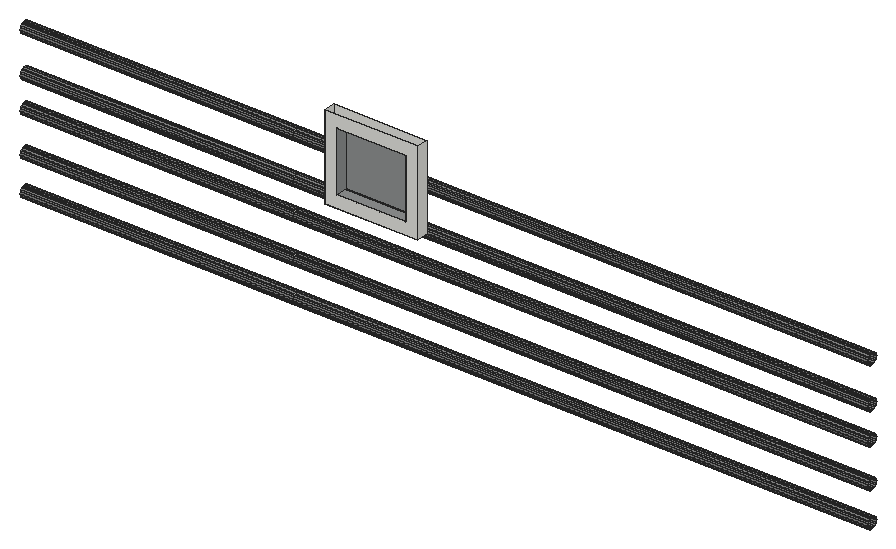
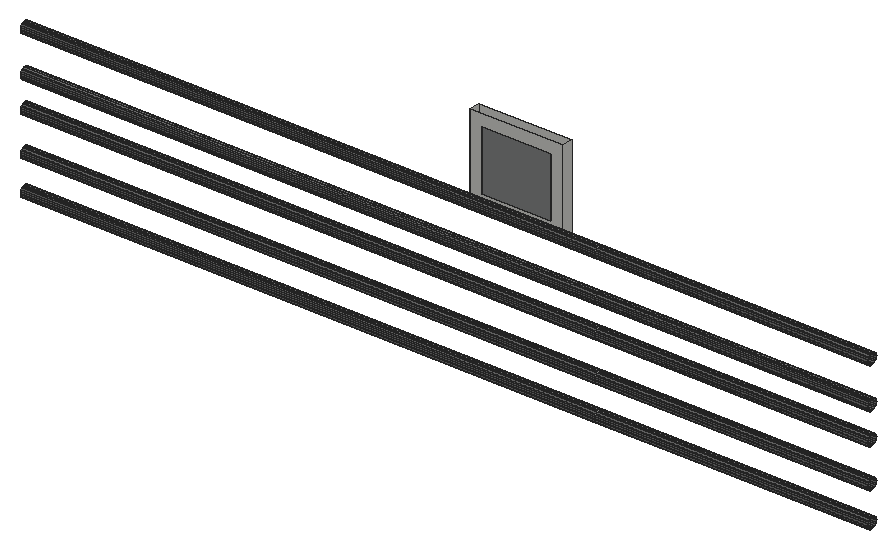
# SketchUp Ruby script. Lengths in inches.
U = 1.inch
M = Sketchup.active_model
def pt(a) = Geom::Point3d.new(a.map { |v| v * U })
def face(e, loops, mat)
  f = e.add_face(loops[0].map { |a| pt(a) })
  loops[1..].each { |l| e.add_face(l.map { |a| pt(a) }).erase! }
  f.material = f.back_material = mat if mat
  f
end
# faces: each face lists its corners as indices into pts; further lists are holes
def faces(e, pts, list, mat = nil) = list.each { |f| face(e, (f[0].is_a?(Array) ? f : [f]).map { |l| l.map { |i| pts[i] } }, mat) }
# xy, xz, yz: faces in a plane at the given z, y or x. An outline is a flat list of corners, or four numbers for a rectangle; further outlines are holes
def ring(l) = l.size == 4 ? [[l[0], l[1]], [l[2], l[1]], [l[2], l[3]], [l[0], l[3]]] : l.each_slice(2).to_a
def flat(e, list, mat, &to3) = list.each { |f| face(e, (f[0].is_a?(Array) ? f : [f]).map { |l| ring(l).map { |u, v| to3.(u, v) } }, mat) }
def xy(e, z, list, mat = nil) = flat(e, list, mat) { |x, y| [x, y, z] }
def xz(e, y, list, mat = nil) = flat(e, list, mat) { |x, z| [x, y, z] }
def yz(e, x, list, mat = nil) = flat(e, list, mat) { |y, z| [x, y, z] }
def lines(e, pts, list) = list.each { |a, b| e.add_line(pt(pts[a]), pt(pts[b])) }
# prism: a flat outline (further loops are holes) pulled along v
def prism(e, loops, v, mat = nil)
  f = face(e, loops, mat); d = Geom::Vector3d.new(v.map { |x| x * U })
  f.pushpull(f.normal.samedirection?(d) ? d.length : -d.length)
end
def box(e, o, s, mat = nil) = prism(e, [[o, [o[0] + s[0], o[1], o[2]], [o[0] + s[0], o[1] + s[1], o[2]], [o[0], o[1] + s[1], o[2]]]], [0, 0, s[2]], mat)
def at(x, y, z, deg = 0) = Geom::Transformation.translation(pt([x, y, z])) * Geom::Transformation.rotation(ORIGIN, Z_AXIS, deg.degrees)
def axes(o, x, y, z) = Geom::Transformation.new([*x, 0, *y, 0, *z, 0, *pt(o).to_a, 1])
def part(name) = M.definitions.add(name)
# library, detail: a bought-in or finely detailed component or shape, given as its bounding box
def library(name, o, s) = part(name).tap { |d| box(d.entities, o, s) }
def detail(e, o, s) = box(e.add_group.entities, o, s)
def put(e, d, t, mat = nil) = e.add_instance(d, t).tap { |i| i.material = mat if mat }
def group(e, t, mat = nil) = e.add_group.tap { |g| g.transformation = t; g.material = mat if mat }.entities
root = M.entities
M.materials.add("[0133_Gray]").color = [128, 128, 128]
M.materials.add("[Blacktop Old 02]").color = [143, 145, 145]
xy(root,158.26,[[226.04,223.92,236.29,225.17]])
xy(root,159.59,[[227.37,223.92,234.96,225.17]],"[Blacktop Old 02]")
xz(root,223.92,[[[226.04,158.26,236.29,167.57],[227.37,159.59,234.96,166.24]]])
xz(root,225.17,[[[226.04,158.26,236.29,167.57],[227.37,159.59,234.96,166.24]]])
xz(root,225.17,[[227.37,159.59,234.96,166.24]],"[Blacktop Old 02]")
yz(root,219.28,[[228.53,143.87,228.6875,143.89,228.84,143.95,228.97,144.05,229.07,144.18,229.13,144.33,229.15,144.49,229.13,144.66,229.07,144.81,228.97,144.9375,228.84,145.04,228.6875,145.1,228.53,145.12,228.36,145.1,228.21,145.04,228.08,144.9375,227.98,144.81,227.92,144.66,227.9,144.49,227.92,144.33,227.98,144.18,228.08,144.05,228.21,143.95,228.36,143.89],[228.53,147.74,228.6875,147.77,228.84,147.83,228.97,147.93,229.07,148.06,229.13,148.21,229.15,148.37,229.13,148.53,229.07,148.68,228.97,148.8125,228.84,148.91,228.6875,148.97,228.53,148.99,228.36,148.97,228.21,148.91,228.08,148.8125,227.98,148.68,227.92,148.53,227.9,148.37,227.92,148.21,227.98,148.06,228.08,147.93,228.21,147.83,228.36,147.77],[228.53,152.12,228.6875,152.14,228.84,152.2,228.97,152.3,229.07,152.43,229.13,152.58,229.15,152.74,229.13,152.91,229.07,153.06,228.97,153.1875,228.84,153.29,228.6875,153.35,228.53,153.37,228.36,153.35,228.21,153.29,228.08,153.1875,227.98,153.06,227.92,152.91,227.9,152.74,227.92,152.58,227.98,152.43,228.08,152.3,228.21,152.2,228.36,152.14],[228.53,155.62,228.6875,155.64,228.84,155.7,228.97,155.8,229.07,155.93,229.13,156.08,229.15,156.24,229.13,156.41,229.07,156.56,228.97,156.6875,228.84,156.79,228.6875,156.85,228.53,156.87,228.36,156.85,228.21,156.79,228.08,156.6875,227.98,156.56,227.92,156.41,227.9,156.24,227.92,156.08,227.98,155.93,228.08,155.8,228.21,155.7,228.36,155.64],[228.53,160.18,228.6875,160.2,228.84,160.27,228.97,160.37,229.07,160.49,229.13,160.65,229.15,160.81,229.13,160.97,229.07,161.12,228.97,161.25,228.84,161.35,228.6875,161.41,228.53,161.43,228.36,161.41,228.21,161.35,228.08,161.25,227.98,161.12,227.92,160.97,227.9,160.81,227.92,160.65,227.98,160.49,228.08,160.37,228.21,160.27,228.36,160.2]])
yz(root,226.04,[[223.92,158.26,225.17,167.57]])
yz(root,227.37,[[223.92,159.59,225.17,166.24]],"[Blacktop Old 02]")
yz(root,234.96,[[223.92,159.59,225.17,166.24]],"[Blacktop Old 02]")
yz(root,236.29,[[223.92,158.26,225.17,167.57]])
p = [[219.28,228.36,143.89],[219.28,228.21,143.95],[189.02,228.21,143.95],[189.02,228.36,143.89],[283.04,228.36,143.89],[283.04,228.21,143.95],
  [219.28,228.53,143.87],[189.02,228.53,143.87],[283.04,228.53,143.87],[219.28,228.6875,143.89],[189.02,228.6875,143.89],[283.04,228.6875,143.89],
  [219.28,228.84,143.95],[189.02,228.84,143.95],[283.04,228.84,143.95],[219.28,228.08,144.05],[189.02,228.08,144.05],[283.04,228.08,144.05],
  [219.28,228.97,144.05],[189.02,228.97,144.05],[283.04,228.97,144.05],[219.28,227.98,144.18],[189.02,227.98,144.18],[283.04,227.98,144.18],
  [219.28,229.07,144.18],[189.02,229.07,144.18],[283.04,229.07,144.18],[219.28,227.92,144.33],[189.02,227.92,144.33],[283.04,227.92,144.33],
  [219.28,229.13,144.33],[189.02,229.13,144.33],[283.04,229.13,144.33],[219.28,227.9,144.49],[189.02,227.9,144.49],[283.04,227.9,144.49],
  [219.28,229.15,144.49],[189.02,229.15,144.49],[283.04,229.15,144.49],[219.28,227.92,144.66],[189.02,227.92,144.66],[283.04,227.92,144.66],
  [219.28,229.13,144.66],[189.02,229.13,144.66],[283.04,229.13,144.66],[219.28,227.98,144.81],[189.02,227.98,144.81],[283.04,227.98,144.81],
  [219.28,229.07,144.81],[189.02,229.07,144.81],[283.04,229.07,144.81],[219.28,228.08,144.9375],[189.02,228.08,144.9375],[283.04,228.08,144.9375],
  [219.28,228.97,144.9375],[189.02,228.97,144.9375],[283.04,228.97,144.9375],[219.28,228.21,145.04],[189.02,228.21,145.04],[283.04,228.21,145.04],
  [219.28,228.84,145.04],[189.02,228.84,145.04],[283.04,228.84,145.04],[219.28,228.36,145.1],[189.02,228.36,145.1],[283.04,228.36,145.1],
  [219.28,228.6875,145.1],[189.02,228.6875,145.1],[283.04,228.6875,145.1],[219.28,228.53,145.12],[189.02,228.53,145.12],[283.04,228.53,145.12],
  [219.28,228.53,147.74],[219.28,228.36,147.77],[189.02,228.36,147.77],[189.02,228.53,147.74],[283.04,228.53,147.74],[283.04,228.36,147.77],
  [219.28,228.6875,147.77],[189.02,228.6875,147.77],[283.04,228.6875,147.77],[219.28,228.21,147.83],[219.28,228.08,147.93],[189.02,228.08,147.93],
  [189.02,228.21,147.83],[283.04,228.21,147.83],[283.04,228.08,147.93],[219.28,228.84,147.83],[189.02,228.84,147.83],[283.04,228.84,147.83],
  [219.28,228.97,147.93],[189.02,228.97,147.93],[283.04,228.97,147.93],[219.28,227.98,148.06],[189.02,227.98,148.06],[283.04,227.98,148.06],
  [219.28,229.07,148.06],[189.02,229.07,148.06],[283.04,229.07,148.06],[219.28,227.92,148.21],[189.02,227.92,148.21],[283.04,227.92,148.21],
  [219.28,229.13,148.21],[189.02,229.13,148.21],[283.04,229.13,148.21],[219.28,227.9,148.37],[189.02,227.9,148.37],[283.04,227.9,148.37],
  [219.28,229.15,148.37],[189.02,229.15,148.37],[283.04,229.15,148.37],[219.28,227.92,148.53],[189.02,227.92,148.53],[283.04,227.92,148.53],
  [219.28,229.13,148.53],[189.02,229.13,148.53],[283.04,229.13,148.53],[219.28,227.98,148.68],[189.02,227.98,148.68],[283.04,227.98,148.68],
  [219.28,229.07,148.68],[189.02,229.07,148.68],[283.04,229.07,148.68],[219.28,228.08,148.8125],[189.02,228.08,148.8125],[283.04,228.08,148.8125],
  [219.28,228.97,148.8125],[189.02,228.97,148.8125],[283.04,228.97,148.8125],[219.28,228.21,148.91],[189.02,228.21,148.91],[283.04,228.21,148.91],
  [219.28,228.84,148.91],[189.02,228.84,148.91],[283.04,228.84,148.91],[219.28,228.36,148.97],[189.02,228.36,148.97],[283.04,228.36,148.97],
  [219.28,228.6875,148.97],[189.02,228.6875,148.97],[283.04,228.6875,148.97],[219.28,228.53,148.99],[189.02,228.53,148.99],[283.04,228.53,148.99],
  [219.28,228.36,152.14],[219.28,228.21,152.2],[189.02,228.21,152.2],[189.02,228.36,152.14],[283.04,228.36,152.14],[283.04,228.21,152.2],
  [219.28,228.53,152.12],[189.02,228.53,152.12],[283.04,228.53,152.12],[219.28,228.6875,152.14],[189.02,228.6875,152.14],[283.04,228.6875,152.14],
  [219.28,228.84,152.2],[189.02,228.84,152.2],[283.04,228.84,152.2],[219.28,228.08,152.3],[189.02,228.08,152.3],[283.04,228.08,152.3],
  [219.28,228.97,152.3],[189.02,228.97,152.3],[283.04,228.97,152.3],[219.28,227.98,152.43],[189.02,227.98,152.43],[283.04,227.98,152.43],
  [219.28,229.07,152.43],[189.02,229.07,152.43],[283.04,229.07,152.43],[219.28,227.92,152.58],[189.02,227.92,152.58],[283.04,227.92,152.58],
  [219.28,229.13,152.58],[189.02,229.13,152.58],[283.04,229.13,152.58],[219.28,227.9,152.74],[189.02,227.9,152.74],[283.04,227.9,152.74],
  [219.28,229.15,152.74],[189.02,229.15,152.74],[283.04,229.15,152.74],[219.28,227.92,152.91],[189.02,227.92,152.91],[283.04,227.92,152.91],
  [219.28,229.13,152.91],[189.02,229.13,152.91],[283.04,229.13,152.91],[219.28,227.98,153.06],[189.02,227.98,153.06],[283.04,227.98,153.06],
  [219.28,229.07,153.06],[189.02,229.07,153.06],[283.04,229.07,153.06],[219.28,228.08,153.1875],[189.02,228.08,153.1875],[283.04,228.08,153.1875],
  [219.28,228.97,153.1875],[189.02,228.97,153.1875],[283.04,228.97,153.1875],[219.28,228.21,153.29],[189.02,228.21,153.29],[283.04,228.21,153.29],
  [219.28,228.84,153.29],[189.02,228.84,153.29],[283.04,228.84,153.29],[219.28,228.36,153.35],[189.02,228.36,153.35],[283.04,228.36,153.35],
  [219.28,228.53,153.37],[189.02,228.53,153.37],[283.04,228.53,153.37],[219.28,228.6875,153.35],[189.02,228.6875,153.35],[283.04,228.6875,153.35],
  [219.28,228.36,155.64],[219.28,228.21,155.7],[189.02,228.21,155.7],[189.02,228.36,155.64],[283.04,228.36,155.64],[283.04,228.21,155.7],
  [219.28,228.53,155.62],[189.02,228.53,155.62],[283.04,228.53,155.62],[219.28,228.6875,155.64],[189.02,228.6875,155.64],[283.04,228.6875,155.64],
  [219.28,228.84,155.7],[189.02,228.84,155.7],[283.04,228.84,155.7],[219.28,228.08,155.8],[189.02,228.08,155.8],[283.04,228.08,155.8],
  [219.28,228.97,155.8],[189.02,228.97,155.8],[283.04,228.97,155.8],[219.28,227.98,155.93],[189.02,227.98,155.93],[283.04,227.98,155.93],
  [219.28,229.07,155.93],[189.02,229.07,155.93],[283.04,229.07,155.93],[219.28,227.92,156.08],[189.02,227.92,156.08],[283.04,227.92,156.08],
  [219.28,229.13,156.08],[189.02,229.13,156.08],[283.04,229.13,156.08],[219.28,227.9,156.24],[189.02,227.9,156.24],[283.04,227.9,156.24],
  [219.28,229.15,156.24],[189.02,229.15,156.24],[283.04,229.15,156.24],[219.28,227.92,156.41],[189.02,227.92,156.41],[283.04,227.92,156.41],
  [219.28,229.13,156.41],[189.02,229.13,156.41],[283.04,229.13,156.41],[219.28,227.98,156.56],[189.02,227.98,156.56],[283.04,227.98,156.56],
  [219.28,229.07,156.56],[189.02,229.07,156.56],[283.04,229.07,156.56],[219.28,228.08,156.6875],[189.02,228.08,156.6875],[283.04,228.08,156.6875],
  [219.28,228.97,156.6875],[189.02,228.97,156.6875],[283.04,228.97,156.6875],[219.28,228.21,156.79],[189.02,228.21,156.79],[283.04,228.21,156.79],
  [219.28,228.84,156.79],[189.02,228.84,156.79],[283.04,228.84,156.79],[219.28,228.36,156.85],[189.02,228.36,156.85],[283.04,228.36,156.85],
  [219.28,228.53,156.87],[189.02,228.53,156.87],[283.04,228.53,156.87],[219.28,228.6875,156.85],[189.02,228.6875,156.85],[283.04,228.6875,156.85],
  [219.28,228.36,160.2],[219.28,228.21,160.27],[189.02,228.21,160.27],[189.02,228.36,160.2],[283.04,228.36,160.2],[283.04,228.21,160.27],
  [219.28,228.53,160.18],[189.02,228.53,160.18],[283.04,228.53,160.18],[219.28,228.6875,160.2],[189.02,228.6875,160.2],[283.04,228.6875,160.2],
  [219.28,228.84,160.27],[189.02,228.84,160.27],[283.04,228.84,160.27],[219.28,228.08,160.37],[189.02,228.08,160.37],[283.04,228.08,160.37],
  [219.28,228.97,160.37],[189.02,228.97,160.37],[283.04,228.97,160.37],[219.28,227.98,160.49],[189.02,227.98,160.49],[283.04,227.98,160.49],
  [219.28,229.07,160.49],[189.02,229.07,160.49],[283.04,229.07,160.49],[219.28,227.92,160.65],[189.02,227.92,160.65],[283.04,227.92,160.65],
  [219.28,229.13,160.65],[189.02,229.13,160.65],[283.04,229.13,160.65],[219.28,227.9,160.81],[189.02,227.9,160.81],[283.04,227.9,160.81],
  [219.28,229.15,160.81],[189.02,229.15,160.81],[283.04,229.15,160.81],[219.28,227.92,160.97],[189.02,227.92,160.97],[283.04,227.92,160.97],
  [219.28,229.13,160.97],[189.02,229.13,160.97],[283.04,229.13,160.97],[219.28,227.98,161.12],[189.02,227.98,161.12],[283.04,227.98,161.12],
  [219.28,229.07,161.12],[189.02,229.07,161.12],[283.04,229.07,161.12],[219.28,228.08,161.25],[189.02,228.08,161.25],[283.04,228.08,161.25],
  [219.28,228.97,161.25],[189.02,228.97,161.25],[283.04,228.97,161.25],[219.28,228.21,161.35],[189.02,228.21,161.35],[283.04,228.21,161.35],
  [219.28,228.84,161.35],[189.02,228.84,161.35],[283.04,228.84,161.35],[219.28,228.36,161.41],[189.02,228.36,161.41],[283.04,228.36,161.41],
  [219.28,228.6875,161.41],[189.02,228.6875,161.41],[283.04,228.6875,161.41],[219.28,228.53,161.43],[189.02,228.53,161.43],[283.04,228.53,161.43]]
faces(root,p,[[0,1,2,3],[1,0,4,5],[6,0,3,7],[0,6,8,4],[9,6,7,10],[6,9,11,8],[12,9,10,13],[9,12,14,11],
  [1,15,16,2],[15,1,5,17],[18,12,13,19],[12,18,20,14],[15,21,22,16],[21,15,17,23],[24,18,19,25],[18,24,26,20],
  [21,27,28,22],[27,21,23,29],[30,24,25,31],[24,30,32,26],[27,33,34,28],[33,27,29,35],[36,30,31,37],[30,36,38,32],
  [33,39,40,34],[39,33,35,41],[42,36,37,43],[36,42,44,38],[39,45,46,40],[45,39,41,47],[48,42,43,49],[42,48,50,44],
  [45,51,52,46],[51,45,47,53],[54,48,49,55],[48,54,56,50],[51,57,58,52],[57,51,53,59],[60,54,55,61],[54,60,62,56],
  [57,63,64,58],[63,57,59,65],[66,60,61,67],[60,66,68,62],[63,69,70,64],[69,63,65,71],[69,66,67,70],[66,69,71,68],
  [72,73,74,75],[73,72,76,77],[78,72,75,79],[72,78,80,76],[81,82,83,84],[82,81,85,86],[73,81,84,74],[81,73,77,85],
  [87,78,79,88],[78,87,89,80],[90,87,88,91],[87,90,92,89],[82,93,94,83],[93,82,86,95],[96,90,91,97],[90,96,98,92],
  [93,99,100,94],[99,93,95,101],[102,96,97,103],[96,102,104,98],[99,105,106,100],[105,99,101,107],[108,102,103,109],[102,108,110,104],
  [105,111,112,106],[111,105,107,113],[114,108,109,115],[108,114,116,110],[111,117,118,112],[117,111,113,119],[120,114,115,121],[114,120,122,116],
  [117,123,124,118],[123,117,119,125],[126,120,121,127],[120,126,128,122],[123,129,130,124],[129,123,125,131],[132,126,127,133],[126,132,134,128],
  [129,135,136,130],[135,129,131,137],[138,132,133,139],[132,138,140,134],[135,141,142,136],[141,135,137,143],[141,138,139,142],[138,141,143,140],
  [144,145,146,147],[145,144,148,149],[150,144,147,151],[144,150,152,148],[153,150,151,154],[150,153,155,152],[156,153,154,157],[153,156,158,155],
  [145,159,160,146],[159,145,149,161],[162,156,157,163],[156,162,164,158],[159,165,166,160],[165,159,161,167],[168,162,163,169],[162,168,170,164],
  [165,171,172,166],[171,165,167,173],[174,168,169,175],[168,174,176,170],[171,177,178,172],[177,171,173,179],[180,174,175,181],[174,180,182,176],
  [177,183,184,178],[183,177,179,185],[186,180,181,187],[180,186,188,182],[183,189,190,184],[189,183,185,191],[192,186,187,193],[186,192,194,188],
  [189,195,196,190],[195,189,191,197],[198,192,193,199],[192,198,200,194],[195,201,202,196],[201,195,197,203],[204,198,199,205],[198,204,206,200],
  [201,207,208,202],[207,201,203,209],[207,210,211,208],[210,207,209,212],[210,213,214,211],[213,210,212,215],[213,204,205,214],[204,213,215,206],
  [216,217,218,219],[217,216,220,221],[222,216,219,223],[216,222,224,220],[225,222,223,226],[222,225,227,224],[228,225,226,229],[225,228,230,227],
  [217,231,232,218],[231,217,221,233],[234,228,229,235],[228,234,236,230],[231,237,238,232],[237,231,233,239],[240,234,235,241],[234,240,242,236],
  [237,243,244,238],[243,237,239,245],[246,240,241,247],[240,246,248,242],[243,249,250,244],[249,243,245,251],[252,246,247,253],[246,252,254,248],
  [249,255,256,250],[255,249,251,257],[258,252,253,259],[252,258,260,254],[255,261,262,256],[261,255,257,263],[264,258,259,265],[258,264,266,260],
  [261,267,268,262],[267,261,263,269],[270,264,265,271],[264,270,272,266],[267,273,274,268],[273,267,269,275],[276,270,271,277],[270,276,278,272],
  [273,279,280,274],[279,273,275,281],[279,282,283,280],[282,279,281,284],[282,285,286,283],[285,282,284,287],[285,276,277,286],[276,285,287,278],
  [288,289,290,291],[289,288,292,293],[294,288,291,295],[288,294,296,292],[297,294,295,298],[294,297,299,296],[300,297,298,301],[297,300,302,299],
  [289,303,304,290],[303,289,293,305],[306,300,301,307],[300,306,308,302],[303,309,310,304],[309,303,305,311],[312,306,307,313],[306,312,314,308],
  [309,315,316,310],[315,309,311,317],[318,312,313,319],[312,318,320,314],[315,321,322,316],[321,315,317,323],[324,318,319,325],[318,324,326,320],
  [321,327,328,322],[327,321,323,329],[330,324,325,331],[324,330,332,326],[327,333,334,328],[333,327,329,335],[336,330,331,337],[330,336,338,332],
  [333,339,340,334],[339,333,335,341],[342,336,337,343],[336,342,344,338],[339,345,346,340],[345,339,341,347],[348,342,343,349],[342,348,350,344],
  [345,351,352,346],[351,345,347,353],[354,348,349,355],[348,354,356,350],[351,357,358,352],[357,351,353,359],[357,354,355,358],[354,357,359,356]],"[0133_Gray]")
